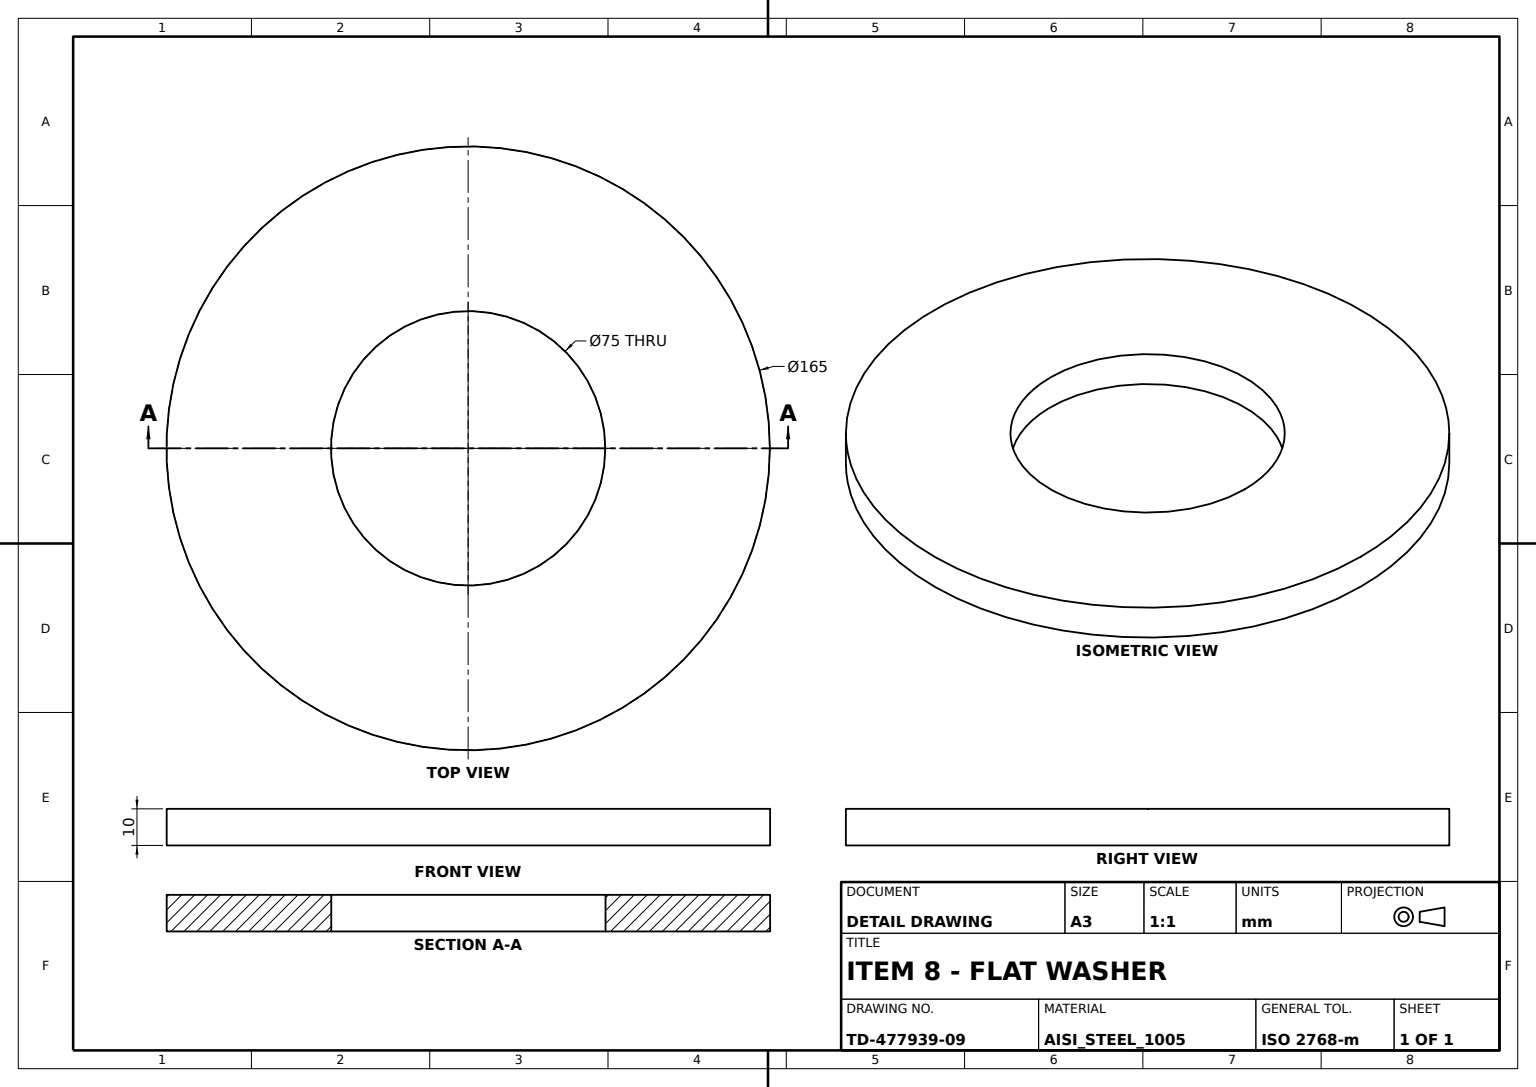
ISO-10303-21;
HEADER;
FILE_DESCRIPTION((''),'2;1');
FILE_NAME('','',(''),(''),'','','');
FILE_SCHEMA(('AUTOMOTIVE_DESIGN'));
ENDSEC;
DATA;
#1=APPLICATION_CONTEXT('');
#2=PRODUCT_CONTEXT('',#1,'mechanical');
#3=PRODUCT('','','',(#2));
#4=PRODUCT_DEFINITION_FORMATION('','',#3);
#5=PRODUCT_DEFINITION_CONTEXT('',#1,'design');
#6=PRODUCT_DEFINITION('','',#4,#5);
#7=PRODUCT_DEFINITION_SHAPE('','',#6);
#8=(LENGTH_UNIT()NAMED_UNIT(*)SI_UNIT(.MILLI.,.METRE.));
#9=(NAMED_UNIT(*)PLANE_ANGLE_UNIT()SI_UNIT($,.RADIAN.));
#10=(NAMED_UNIT(*)SI_UNIT($,.STERADIAN.)SOLID_ANGLE_UNIT());
#11=UNCERTAINTY_MEASURE_WITH_UNIT(LENGTH_MEASURE(0.005),#8,'distance_accuracy_value','');
#12=(GEOMETRIC_REPRESENTATION_CONTEXT(3)GLOBAL_UNCERTAINTY_ASSIGNED_CONTEXT((#11))GLOBAL_UNIT_ASSIGNED_CONTEXT((#8,#9,#10))REPRESENTATION_CONTEXT('',''));
#13=CARTESIAN_POINT('',(37.5,0.,10.));
#14=VERTEX_POINT('',#13);
#15=CARTESIAN_POINT('',(0.,0.,10.));
#16=DIRECTION('',(0.,0.,-1.));
#17=DIRECTION('',(1.,0.,0.));
#18=AXIS2_PLACEMENT_3D('',#15,#16,#17);
#19=CIRCLE('',#18,37.5);
#20=EDGE_CURVE('',#14,#14,#19,.T.);
#21=ORIENTED_EDGE('',*,*,#20,.T.);
#22=EDGE_LOOP('',(#21));
#23=FACE_BOUND('',#22,.T.);
#24=CARTESIAN_POINT('',(82.5,0.,10.));
#25=VERTEX_POINT('',#24);
#26=CIRCLE('',#18,82.5);
#27=EDGE_CURVE('',#25,#25,#26,.T.);
#28=ORIENTED_EDGE('',*,*,#27,.F.);
#29=EDGE_LOOP('',(#28));
#30=FACE_BOUND('',#29,.T.);
#31=DIRECTION('',(-1.,0.,0.));
#32=AXIS2_PLACEMENT_3D('',#15,#16,#31);
#33=PLANE('',#32);
#34=ADVANCED_FACE('',(#23,#30),#33,.F.);
#35=CARTESIAN_POINT('',(82.5,0.,0.));
#36=VERTEX_POINT('',#35);
#37=CARTESIAN_POINT('',(0.,0.,0.));
#38=AXIS2_PLACEMENT_3D('',#37,#16,#17);
#39=CIRCLE('',#38,82.5);
#40=EDGE_CURVE('',#36,#36,#39,.T.);
#41=ORIENTED_EDGE('',*,*,#40,.F.);
#42=EDGE_LOOP('',(#41));
#43=FACE_BOUND('',#42,.T.);
#44=ORIENTED_EDGE('',*,*,#27,.T.);
#45=EDGE_LOOP('',(#44));
#46=FACE_BOUND('',#45,.T.);
#47=CYLINDRICAL_SURFACE('',#32,82.5);
#48=ADVANCED_FACE('',(#43,#46),#47,.T.);
#49=ORIENTED_EDGE('',*,*,#20,.F.);
#50=EDGE_LOOP('',(#49));
#51=FACE_BOUND('',#50,.T.);
#52=CARTESIAN_POINT('',(37.5,0.,0.));
#53=VERTEX_POINT('',#52);
#54=CIRCLE('',#38,37.5);
#55=EDGE_CURVE('',#53,#53,#54,.T.);
#56=ORIENTED_EDGE('',*,*,#55,.T.);
#57=EDGE_LOOP('',(#56));
#58=FACE_BOUND('',#57,.T.);
#59=CYLINDRICAL_SURFACE('',#32,37.5);
#60=ADVANCED_FACE('',(#51,#58),#59,.F.);
#61=ORIENTED_EDGE('',*,*,#40,.T.);
#62=EDGE_LOOP('',(#61));
#63=FACE_BOUND('',#62,.T.);
#64=ORIENTED_EDGE('',*,*,#55,.F.);
#65=EDGE_LOOP('',(#64));
#66=FACE_BOUND('',#65,.T.);
#67=AXIS2_PLACEMENT_3D('',#37,#16,#31);
#68=PLANE('',#67);
#69=ADVANCED_FACE('',(#63,#66),#68,.T.);
#70=CLOSED_SHELL('',(#34,#48,#60,#69));
#71=MANIFOLD_SOLID_BREP('',#70);
#72=ADVANCED_BREP_SHAPE_REPRESENTATION('',(#71),#12);
#73=SHAPE_DEFINITION_REPRESENTATION(#7,#72);
ENDSEC;
END-ISO-10303-21;
